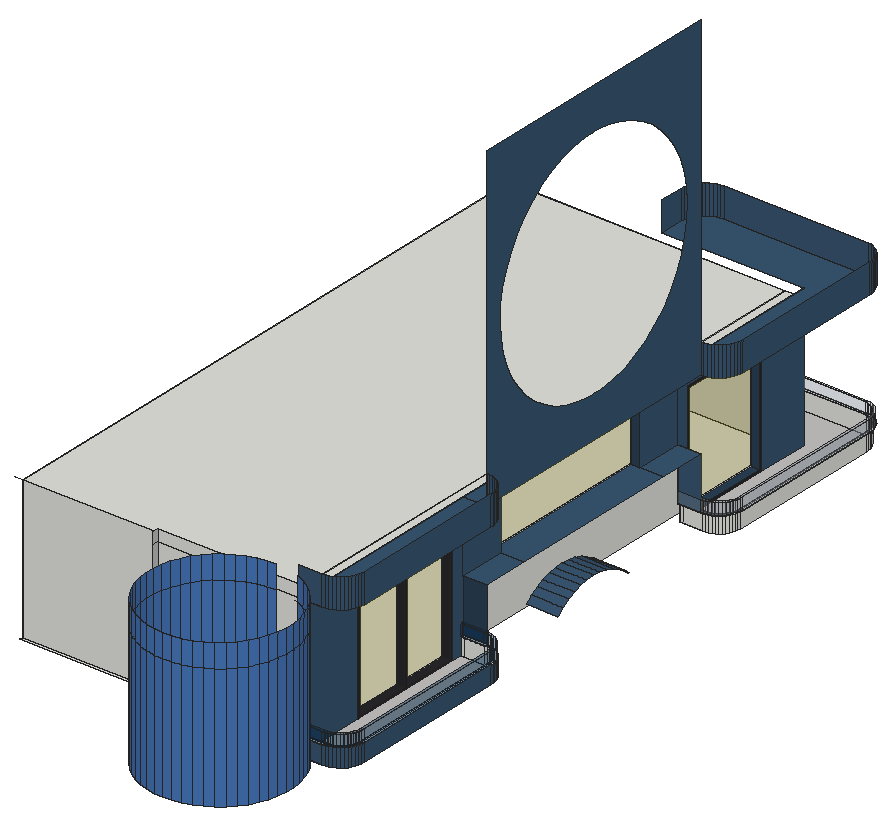
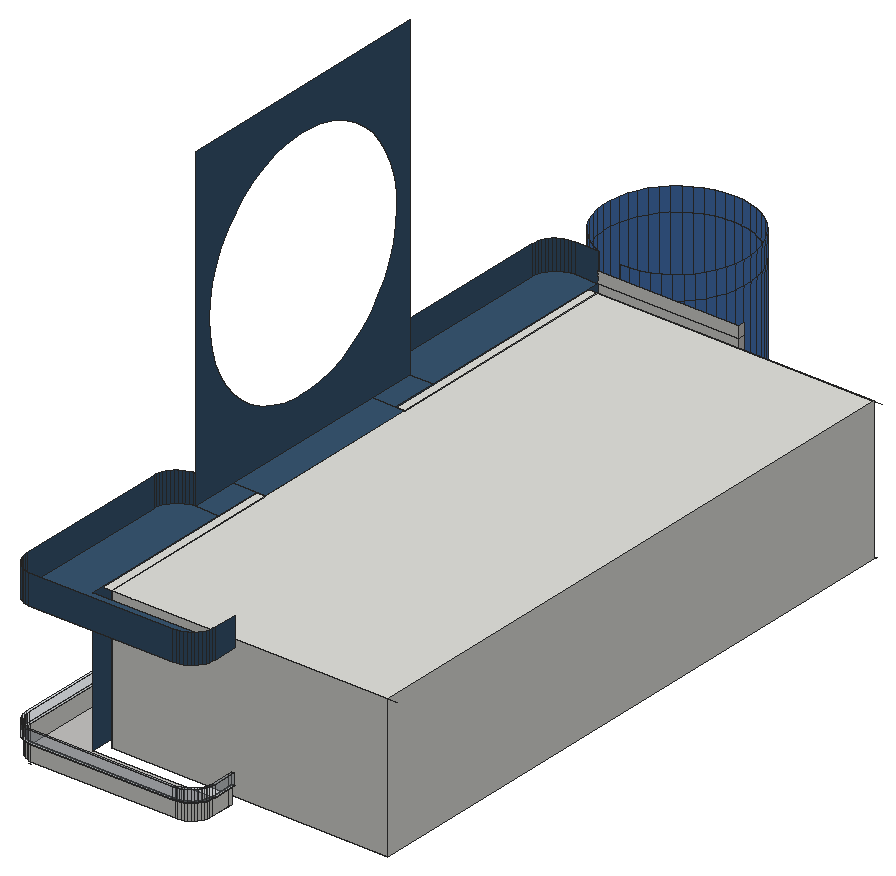
# SketchUp Ruby script. Lengths in inches.
U = 1.inch
M = Sketchup.active_model
def pt(a) = Geom::Point3d.new(a.map { |v| v * U })
def face(e, loops, mat)
  f = e.add_face(loops[0].map { |a| pt(a) })
  loops[1..].each { |l| e.add_face(l.map { |a| pt(a) }).erase! }
  f.material = f.back_material = mat if mat
  f
end
# faces: each face lists its corners as indices into pts; further lists are holes
def faces(e, pts, list, mat = nil) = list.each { |f| face(e, (f[0].is_a?(Array) ? f : [f]).map { |l| l.map { |i| pts[i] } }, mat) }
# xy, xz, yz: faces in a plane at the given z, y or x. An outline is a flat list of corners, or four numbers for a rectangle; further outlines are holes
def ring(l) = l.size == 4 ? [[l[0], l[1]], [l[2], l[1]], [l[2], l[3]], [l[0], l[3]]] : l.each_slice(2).to_a
def flat(e, list, mat, &to3) = list.each { |f| face(e, (f[0].is_a?(Array) ? f : [f]).map { |l| ring(l).map { |u, v| to3.(u, v) } }, mat) }
def xy(e, z, list, mat = nil) = flat(e, list, mat) { |x, y| [x, y, z] }
def xz(e, y, list, mat = nil) = flat(e, list, mat) { |x, z| [x, y, z] }
def yz(e, x, list, mat = nil) = flat(e, list, mat) { |y, z| [x, y, z] }
def lines(e, pts, list) = list.each { |a, b| e.add_line(pt(pts[a]), pt(pts[b])) }
# prism: a flat outline (further loops are holes) pulled along v
def prism(e, loops, v, mat = nil)
  f = face(e, loops, mat); d = Geom::Vector3d.new(v.map { |x| x * U })
  f.pushpull(f.normal.samedirection?(d) ? d.length : -d.length)
end
def box(e, o, s, mat = nil) = prism(e, [[o, [o[0] + s[0], o[1], o[2]], [o[0] + s[0], o[1] + s[1], o[2]], [o[0], o[1] + s[1], o[2]]]], [0, 0, s[2]], mat)
def at(x, y, z, deg = 0) = Geom::Transformation.translation(pt([x, y, z])) * Geom::Transformation.rotation(ORIGIN, Z_AXIS, deg.degrees)
def axes(o, x, y, z) = Geom::Transformation.new([*x, 0, *y, 0, *z, 0, *pt(o).to_a, 1])
def part(name) = M.definitions.add(name)
# library, detail: a bought-in or finely detailed component or shape, given as its bounding box
def library(name, o, s) = part(name).tap { |d| box(d.entities, o, s) }
def detail(e, o, s) = box(e.add_group.entities, o, s)
def put(e, d, t, mat = nil) = e.add_instance(d, t).tap { |i| i.material = mat if mat }
def group(e, t, mat = nil) = e.add_group.tap { |g| g.transformation = t; g.material = mat if mat }.entities
root = M.entities
M.materials.add("Carpet_01_1K").color = [196, 195, 193]
M.materials.add("Carpet_04_1K").color = [56, 85, 112]
M.materials.add("Carpet_04_1K1").color = [43, 65, 85]
M.materials.add("Glass_Basic_01").color = [186, 175, 28]
M.materials["Glass_Basic_01"].alpha = 0.25
M.materials.add("Glass_Basic_1").color = [0, 47, 91]
M.materials["Glass_Basic_1"].alpha = 0.25
M.materials.add("Glass_Basic_2").color = [161, 173, 186]
M.materials["Glass_Basic_2"].alpha = 0.25
M.materials.add("Glass_Mirror_01").color = [71, 118, 185]
M.materials.add("ThomThom - Buttons2").color = [40, 40, 43]
c1 = part("Group\#1")
prism(c1.entities,[[[0,206.04,0],[0,209.04,0],[24,209.04,0],[24.001,209.04,0],[27.133,208.835,0],[30.212,208.222,0],[33.184,207.213,0],[36,205.825,0],[38.61,204.081,0],[40.971,202.011,0],[43.04,199.65,0],[44.785,197.04,0],[46.173,194.224,0],[47.182,191.252,0],[47.795,188.173,0],[48,185.04,0],[48,24,0],[47.795,20.867,0],[47.182,17.788,0],[46.602,16.08,0],[46.173,14.816,0],[44.785,12,0],[43.04,9.39,0],[40.971,7.029,0],[38.61,4.96,0],[36,3.215,0],[33.184,1.827,0],[30.212,0.818,0],[27.133,0.205,0],[24,0,0],[0,0,0],[0,3,0],[3,3,0],[24,3,0],[26.741,3.18,0],[29.435,3.716,0],[32.036,4.599,0],[34.5,5.814,0],[36.784,7.34,0],[38.849,9.151,0],[40.66,11.216,0],[42.187,13.5,0],[43.401,15.964,0],[44.284,18.565,0],[44.82,21.259,0],[45,24,0],[45,185.04,0],[44.82,187.781,0],[44.284,190.475,0],[43.401,193.076,0],[42.187,195.54,0],[40.66,197.824,0],[38.849,199.889,0],[36.784,201.701,0],[34.5,203.227,0],[32.036,204.442,0],[29.435,205.325,0],[26.741,205.86,0],[24,206.04,0],[3,206.04,0]]],[0,0,12])
c2 = part("Group\#2")
prism(c2.entities,[[[147,3,0],[168,3,0],[170.74,3.18,0],[173.44,3.72,0],[176.04,4.6,0],[178.5,5.8125,0],[180.78,7.34,0],[182.85,9.15,0],[184.66,11.22,0],[186.1875,13.5,0],[187.4,15.96,0],[188.28,18.56,0],[188.82,21.26,0],[189,24,0],[189,184.94,0],[188.8125,187.78,0],[188.28,190.47,0],[187.4,193.07,0],[186.18,195.54,0],[184.66,197.82,0],[182.84,199.88,0],[180.78,201.7,0],[178.5,203.22,0],[176.03,204.4375,0],[173.43,205.32,0],[171.01,205.8,0],[24,205.8,0],[21.26,205.62,0],[18.56,205.08,0],[15.96,204.2,0],[13.5,202.99,0],[11.22,201.46,0],[9.15,199.65,0],[7.34,197.58,0],[5.8125,195.3,0],[4.6,192.84,0],[3.72,190.24,0],[3.18,187.54,0],[3,184.8,0],[3,163.8,0],[3,160.8,0],[0,160.8,0],[0,184.8,0],[0.21,187.93,0],[0.82,191.01,0],[1.83,193.98,0],[3.22,196.8,0],[4.96,199.41,0],[7.03,201.77,0],[9.39,203.84,0],[12,205.58,0],[14.82,206.97,0],[17.79,207.98,0],[20.87,208.59,0],[24,208.8,0],[171.31,208.8,0],[174.21,208.22,0],[177.18,207.21,0],[180,205.82,0],[182.61,204.08,0],[184.97,202.01,0],[187.04,199.65,0],[188.78,197.04,0],[190.17,194.22,0],[191.18,191.25,0],[191.79,188.17,0],[192,185.04,0],[192,24,0],[191.79,20.87,0],[191.18,17.79,0],[190.17,14.82,0],[188.78,12,0],[187.04,9.39,0],[184.97,7.03,0],[182.61,4.96,0],[180,3.22,0],[177.18,1.83,0],[174.21,0.82,0],[171.13,0.21,0],[168,0,0],[144,0,0],[144,3,0]]],[0,0,12])
xy(root,461.77,[[330.57,155.5,354.57,155.5,357.71,155.71,360.79,156.32,363.76,157.33,366.57,158.72,369.19,160.46,371.55,162.53,373.62,164.89,375.36,167.5,376.75,170.32,377.76,173.29,378.37,176.37,378.57,179.5,378.57,340.54,378.37,343.67,377.76,346.75,376.75,349.73,375.36,352.54,373.62,355.15,371.55,357.51,369.19,359.58,366.57,361.33,363.76,362.71,360.79,363.72,357.71,364.34,354.58,364.54,330.57,364.54,330.57,361.54,354.57,361.54,357.32,361.36,360.01,360.83,362.61,359.94,365.07,358.73,367.36,357.2,369.42,355.39,371.24,353.33,372.76,351.04,373.98,348.58,374.86,345.98,375.4,343.28,375.57,340.54,375.57,179.5,375.4,176.76,374.86,174.07,373.98,171.46,372.76,169,371.24,166.72,369.42,164.65,367.36,162.84,365.07,161.31,362.61,160.1,360.01,159.22,357.32,158.68,354.57,158.5,330.57,158.5]])
xy(root,462,[[39.57,164.5,321.57,167.5625],[39.57,167.5625,321.57,786.64]])
xy(root,462,[[330.57,158.5,354.57,158.5,357.32,158.68,360.01,159.22,362.61,160.1,365.07,161.31,367.36,162.84,369.42,164.65,371.24,166.72,372.76,169,373.98,171.46,374.86,174.07,375.4,176.76,375.57,179.5,375.57,340.54,375.4,343.28,374.86,345.98,373.98,348.58,372.76,351.04,371.24,353.33,369.42,355.39,367.36,357.2,365.07,358.73,362.61,359.94,360.01,360.83,357.32,361.36,354.57,361.54,330.57,361.54],[330.57,640.9,354.57,640.9,357.32,641.08,360.01,641.62,362.61,642.5,365.07,643.71,367.36,645.24,369.42,647.05,371.24,649.12,372.76,651.4,373.98,653.86,374.86,656.47,375.4,659.16,375.57,661.9,375.57,822.84,375.39,825.68,374.85,828.375,373.97,830.97,372.76,833.4375,371.23,835.72,369.42,837.79,367.36,839.6,365.07,841.12,362.61,842.34,360.01,843.22,357.59,843.7,210.57,843.7,207.83,843.52,205.14,842.99,202.54,842.1,200.07,840.89,197.79,839.36,195.73,837.55,193.91,835.48,192.39,833.2,191.17,830.74,190.29,828.14,189.75,825.44,189.57,822.7,189.57,798.7,330.57,798.7]],"Carpet_01_1K")
xy(root,463.77,[[321.57,233.15,330.57,291.15],[321.57,293.15,330.57,349.15]],"ThomThom - Buttons2")
xy(root,465,[[321.57,652.9,330.57,742.9]],"Carpet_04_1K1")
xy(root,480,[[330.57,155.5,354.57,155.5,357.71,155.71,360.79,156.32,363.76,157.33,366.57,158.72,369.19,160.46,371.55,162.53,373.62,164.89,375.36,167.5,376.75,170.32,377.76,173.29,378.37,176.37,378.57,179.5,378.57,340.54,378.37,343.67,377.76,346.75,376.75,349.73,375.36,352.54,373.62,355.15,371.55,357.51,369.19,359.58,366.57,361.33,363.76,362.71,360.79,363.72,357.71,364.34,354.58,364.54,330.57,364.54,330.57,361.54,354.57,361.54,357.32,361.36,360.01,360.83,362.61,359.94,365.07,358.73,367.36,357.2,369.42,355.39,371.24,353.33,372.76,351.04,373.98,348.58,374.86,345.98,375.4,343.28,375.57,340.54,375.57,179.5,375.4,176.76,374.86,174.07,373.98,171.46,372.76,169,371.24,166.72,369.42,164.65,367.36,162.84,365.07,161.31,362.61,160.1,360.01,159.22,357.32,158.68,354.57,158.5,330.57,158.5],[330.57,637.9,354.57,637.9,357.71,638.11,360.79,638.72,363.76,639.73,366.57,641.12,369.19,642.86,371.55,644.93,373.62,647.29,375.36,649.9,376.75,652.72,377.76,655.6875,378.37,658.77,378.57,661.9,378.57,822.94,378.37,826.07,377.76,829.15,376.75,832.125,375.36,834.94,373.62,837.55,371.55,839.91,369.19,841.98,366.57,843.73,363.76,845.11,360.79,846.12,357.88,846.7,210.57,846.7,207.44,846.5,204.36,845.88,201.39,844.875,198.57,843.49,195.96,841.74,193.6,839.67,191.53,837.3125,189.79,834.7,188.4,831.89,187.39,828.91,186.78,825.83,186.57,822.7,186.57,798.7,189.57,798.7,189.57,822.7,189.75,825.44,190.29,828.14,191.17,830.74,192.39,833.2,193.91,835.48,195.73,837.55,197.79,839.36,200.07,840.89,202.54,842.1,205.14,842.99,207.83,843.52,210.57,843.7,357.59,843.7,360.01,843.22,362.61,842.34,365.07,841.12,367.36,839.6,369.42,837.79,371.23,835.72,372.76,833.4375,373.97,830.97,374.85,828.375,375.39,825.68,375.57,822.84,375.57,661.9,375.4,659.16,374.86,656.47,373.98,653.86,372.76,651.4,371.24,649.12,369.42,647.05,367.36,645.24,365.07,643.71,362.61,642.5,360.01,641.62,357.32,641.08,354.57,640.9,330.57,640.9]])
xy(root,483,[[322.57,501.22,354.57,501.27]],"Carpet_04_1K")
xy(root,534,[[330.57,364.54,354.57,412.54],[321.57,412.54,354.57,589.9],[330.57,589.9,354.57,637.9]],"Carpet_04_1K")
xy(root,579,[[321.57,652.9,330.57,742.9]],"Carpet_04_1K1")
xy(root,585.77,[[321.57,233.15,330.57,291.15],[321.57,293.15,330.57,349.15]],"ThomThom - Buttons2")
xy(root,606,[[39.57,167.5625,321.57,786.64],[321.57,167.5625,330.57,412.54],[321.57,589.9,330.57,786.64]])
xy(root,606,[[330.57,155.5,330.57,364.54,354.57,364.54,357.71,364.34,360.79,363.72,363.76,362.71,366.57,361.33,369.19,359.58,371.55,357.51,373.62,355.15,375.36,352.54,376.75,349.73,377.76,346.75,378.37,343.67,378.57,340.54,378.57,179.5,378.37,176.37,377.76,173.29,376.75,170.32,375.36,167.5,373.62,164.89,371.55,162.53,369.19,160.46,366.57,158.72,363.76,157.33,360.79,156.32,357.71,155.71,354.57,155.5],[330.57,364.54,354.57,412.54],[321.57,412.54,354.57,589.9],[330.57,589.9,354.57,637.9],[330.57,637.9,330.57,798.7,186.57,798.7,186.57,822.7,186.78,825.83,187.39,828.91,188.4,831.89,189.79,834.7,191.53,837.3125,193.6,839.67,195.96,841.74,198.57,843.49,201.39,844.875,204.36,845.88,207.44,846.5,210.57,846.7,357.88,846.7,360.79,846.12,363.76,845.11,366.57,843.73,369.19,841.98,371.55,839.91,373.62,837.55,375.36,834.94,376.75,832.125,377.76,829.15,378.37,826.07,378.57,822.94,378.57,661.9,378.37,658.77,377.76,655.6875,376.75,652.72,375.36,649.9,373.62,647.29,371.55,644.93,369.19,642.86,366.57,641.12,363.76,639.73,360.79,638.72,357.71,638.11,354.57,637.9]],"Carpet_04_1K")
xz(root,155.5,[[186.57,462,330.57,606],[186.57,606,330.57,618]])
xz(root,155.5,[[330.57,461.77,354.57,480],[330.57,606,354.57,636]],"Carpet_04_1K")
xz(root,158.5,[[330.57,462,333.57,480],[333.57,462,354.57,480]])
xz(root,167.5625,[[39.57,462,321.57,606]])
xz(root,233.15,[[321.57,463.77,330.57,585.77]],"ThomThom - Buttons2")
xz(root,291.15,[[321.57,463.77,330.57,585.77]],"ThomThom - Buttons2")
xz(root,293.15,[[321.57,463.77,330.57,585.77]])
xz(root,349.15,[[321.57,463.77,330.57,585.77]],"ThomThom - Buttons2")
xz(root,361.54,[[330.57,462,333.57,480],[333.57,462,354.57,480]])
xz(root,364.54,[[354.57,461.77,354.58,480]])
xz(root,364.54,[[330.57,480,354.57,534]],"Carpet_04_1K1")
xz(root,412.54,[[321.57,534,330.57,606]])
xz(root,589.9,[[321.57,534,330.57,606]],"Carpet_04_1K1")
xz(root,637.9,[[330.57,480,354.57,534]],"Carpet_04_1K")
xz(root,640.9,[[330.57,462,333.57,480],[333.57,462,354.57,480]])
xz(root,652.9,[[321.57,465,330.57,579]])
xz(root,742.9,[[321.57,465,330.57,579]],"Carpet_04_1K1")
xz(root,786.64,[[39.57,462,321.57,606]])
xz(root,843.7,[[210.57,462,357.59,480]])
xz(root,846.7,[[210.57,606,357.88,636]],"Carpet_04_1K")
yz(root,39.57,[[167.5625,462,786.64,606]])
yz(root,186.57,[[149.51,462,155.5,606],[149.51,606,155.5,618]],"Carpet_01_1K")
yz(root,186.57,[[798.7,606,822.7,636]],"Carpet_04_1K")
yz(root,189.57,[[798.7,462,801.7,480],[801.7,462,822.7,480]])
yz(root,236.92,[[77.22,480,86.26,606],[77.22,606,86.26,630]],"Glass_Mirror_01")
yz(root,321.57,[[[167.5625,462,167.5625,606,412.54,606,412.54,534,589.9,534,589.9,606,786.64,606,786.64,462],[652.9,465,742.9,579],[233.15,463.77,291.15,585.77],[293.15,463.77,349.15,585.77]]])
yz(root,321.57,[[233.15,463.77,291.15,585.77],[293.15,463.77,349.15,585.77],[652.9,465,742.9,579],[412.54,534,589.9,606]],"Glass_Basic_01")
yz(root,330.57,[[231.15,461.77,351.15,462]])
yz(root,330.57,[[158.5,462,231.15,462,231.15,587.77,351.15,587.77,351.15,462,361.54,462,361.54,480,364.54,480,364.54,606,155.5,606,155.5,480,158.5,480],[640.9,462,649.9,462,649.9,582,745.9,582,745.9,462,798.7,462,798.7,606,637.9,606,637.9,480,640.9,480],[364.54,534,412.54,606],[589.9,534,637.9,606]],"Carpet_04_1K")
yz(root,330.57,[[[231.15,462,351.15,587.77],[233.15,463.77,233.15,585.77,349.15,585.77,349.15,463.77,293.15,463.77,293.15,585.77,291.15,585.77,291.15,463.77]],[649.9,462,652.9,462,652.9,579,745.9,579,745.9,582,649.9,582],[652.9,462,745.9,462,745.9,579,742.9,579,742.9,465,652.9,465]],"ThomThom - Buttons2")
yz(root,354.57,[[[364.54,606,637.9,930],[495.8125,648.12,480.83,649.75,466.17,653.23,452.0625,658.53,438.73,665.56,426.38,674.2,415.22,684.32,405.41,695.75,397.11,708.33,390.45,721.85,385.54,736.1,382.45,750.85,381.24,765.87,381.92,780.93,384.48,795.78,388.88,810.1875,395.06,823.9375,402.9,836.8,412.3,848.58,423.1,859.09,435.13,868.16,448.21,875.66,462.12,881.45,476.65,885.46,491.5625,887.61,501.22,887.78,506.63,887.88,521.61,886.25,536.27,882.77,550.38,877.47,563.71,870.44,576.06,861.8,587.23,851.68,597.04,840.25,605.34,827.67,611.99,814.15,616.9,799.9,619.99,785.15,621.2,770.13,620.52,755.07,617.96,740.22,613.56,725.8125,607.39,712.0625,599.54,699.2,590.14,687.42,579.34,676.91,567.31,667.84,554.23,660.34,540.32,654.55,525.79,650.54,510.88,648.39,501.22,648.22]]],"Carpet_04_1K")
yz(root,375.57,[[179.5,462,340.54,480],[661.9,462,822.84,480]])
yz(root,378.57,[[179.5,461.77,340.54,480],[179.5,606,340.54,636],[661.9,606,822.94,636]],"Carpet_04_1K")
yz(root,380.64,[[77.22,480,86.26,606],[77.22,606,86.26,630]],"Glass_Mirror_01")
p = [[354.57,155.5,480],[354.57,155.5,461.77],[357.71,155.71,461.77],[357.71,155.71,480],[360.79,156.32,461.77],[360.79,156.32,480],
  [363.76,157.33,461.77],[363.76,157.33,480],[366.57,158.72,461.77],[366.57,158.72,480],[369.19,160.46,461.77],[369.19,160.46,480],
  [371.55,162.53,461.77],[371.55,162.53,480],[373.62,164.89,461.77],[373.62,164.89,480],[375.36,167.5,461.77],[375.36,167.5,480],
  [376.75,170.32,461.77],[376.75,170.32,480],[377.76,173.29,461.77],[377.76,173.29,480],[378.37,176.37,461.77],[378.37,176.37,480],
  [378.57,179.5,461.77],[378.57,179.5,480],[378.57,340.54,480],[378.57,340.54,461.77],[378.37,343.67,461.77],[378.37,343.67,480],
  [377.76,346.75,461.77],[377.76,346.75,480],[376.75,349.73,461.77],[376.75,349.73,480],[375.36,352.54,461.77],[375.36,352.54,480],
  [373.62,355.15,461.77],[373.62,355.15,480],[371.55,357.51,461.77],[371.55,357.51,480],[369.19,359.58,461.77],[369.19,359.58,480],
  [366.57,361.33,461.77],[366.57,361.33,480],[363.76,362.71,461.77],[363.76,362.71,480],[360.79,363.72,461.77],[360.79,363.72,480],
  [357.71,364.34,461.77],[357.71,364.34,480],[354.58,364.54,461.77],[354.58,364.54,480],[357.32,158.68,462],[354.57,158.5,462],
  [354.57,158.5,480],[357.32,158.68,480],[360.01,159.22,462],[360.01,159.22,480],[362.61,160.1,462],[362.61,160.1,480],
  [365.07,161.31,462],[365.07,161.31,480],[367.36,162.84,462],[367.36,162.84,480],[369.42,164.65,462],[369.42,164.65,480],
  [371.24,166.72,462],[371.24,166.72,480],[372.76,169,462],[372.76,169,480],[373.98,171.46,462],[373.98,171.46,480],
  [374.86,174.07,462],[374.86,174.07,480],[375.4,176.76,462],[375.4,176.76,480],[375.57,179.5,462],[375.57,179.5,480],
  [375.4,343.28,462],[375.57,340.54,462],[375.57,340.54,480],[375.4,343.28,480],[374.86,345.98,462],[374.86,345.98,480],
  [373.98,348.58,462],[373.98,348.58,480],[372.76,351.04,462],[372.76,351.04,480],[371.24,353.33,462],[371.24,353.33,480],
  [369.42,355.39,462],[369.42,355.39,480],[367.36,357.2,462],[367.36,357.2,480],[365.07,358.73,462],[365.07,358.73,480],
  [362.61,359.94,462],[362.61,359.94,480],[360.01,360.83,462],[360.01,360.83,480],[357.32,361.36,462],[357.32,361.36,480],
  [354.57,361.54,462],[354.57,361.54,480],[357.32,641.08,462],[354.57,640.9,462],[354.57,640.9,480],[357.32,641.08,480],
  [360.01,641.62,462],[360.01,641.62,480],[362.61,642.5,462],[362.61,642.5,480],[365.07,643.71,462],[365.07,643.71,480],
  [367.36,645.24,462],[367.36,645.24,480],[369.42,647.05,462],[369.42,647.05,480],[371.24,649.12,462],[371.24,649.12,480],
  [372.76,651.4,462],[372.76,651.4,480],[373.98,653.86,462],[373.98,653.86,480],[374.86,656.47,462],[374.86,656.47,480],
  [375.4,659.16,462],[375.4,659.16,480],[375.57,661.9,462],[375.57,661.9,480],[189.57,822.7,462],[189.75,825.44,462],
  [189.75,825.44,480],[189.57,822.7,480],[375.39,825.68,462],[375.57,822.84,462],[375.57,822.84,480],[375.39,825.68,480],
  [190.29,828.14,462],[190.29,828.14,480],[374.85,828.375,462],[374.85,828.375,480],[191.17,830.74,462],[191.17,830.74,480],
  [373.97,830.97,462],[373.97,830.97,480],[192.39,833.2,462],[192.39,833.2,480],[372.76,833.4375,462],[372.76,833.4375,480],
  [193.91,835.48,462],[193.91,835.48,480],[371.23,835.72,462],[371.23,835.72,480],[195.73,837.55,462],[195.73,837.55,480],
  [369.42,837.79,462],[369.42,837.79,480],[197.79,839.36,462],[197.79,839.36,480],[367.36,839.6,462],[367.36,839.6,480],
  [200.07,840.89,462],[200.07,840.89,480],[365.07,841.12,462],[365.07,841.12,480],[202.54,842.1,462],[202.54,842.1,480],
  [362.61,842.34,462],[362.61,842.34,480],[205.14,842.99,462],[205.14,842.99,480],[360.01,843.22,462],[360.01,843.22,480],
  [207.83,843.52,462],[207.83,843.52,480],[357.59,843.7,462],[357.59,843.7,480],[210.57,843.7,462],[210.57,843.7,480],
  [322.57,462.47,470.43],[354.57,462.47,470.43],[354.57,456.08,465.15],[322.57,456.08,465.15],[322.57,546.4375,465.08],[354.57,546.4375,465.08],
  [354.57,540.06,470.36],[322.57,540.06,470.36],[322.57,469.47,474.86],[354.57,469.47,474.86],[354.57,533.0625,474.8125],[322.57,533.0625,474.8125],
  [354.57,525.57,478.35],[322.57,525.57,478.35],[322.57,476.97,478.38],[354.57,476.97,478.38],[354.57,517.68,480.91],[322.57,517.68,480.91],
  [322.57,484.86,480.9375],[354.57,484.86,480.9375],[299.76,10.31,606],[299.76,10.31,480],[308.78,9.74,480],[308.78,9.74,606],
  [317.8,10.31,480],[317.8,10.31,606],[290.875,12,606],[290.875,12,480],[326.6875,12,480],[326.6875,12,606],
  [282.28,14.79,606],[282.28,14.79,480],[335.29,14.79,480],[335.29,14.79,606],[274.09,18.64,606],[274.09,18.64,480],
  [343.47,18.64,480],[343.47,18.64,606],[266.46,23.49,606],[266.46,23.49,480],[351.1,23.49,480],[351.1,23.49,606],
  [259.49,29.25,606],[259.49,29.25,480],[358.07,29.25,480],[358.07,29.25,606],[253.3,35.84,606],[253.3,35.84,480],
  [364.26,35.84,480],[364.26,35.84,606],[247.99,43.16,606],[247.99,43.16,480],[369.57,43.16,480],[369.57,43.16,606],
  [243.63,51.08,606],[243.63,51.08,480],[373.93,51.08,480],[373.93,51.08,606],[240.3,59.49,606],[240.3,59.49,480],
  [377.26,59.49,480],[377.26,59.49,606],[238.06,68.25,606],[238.06,68.25,480],[379.51,68.25,480],[379.51,68.25,606],
  [236.92,77.22,606],[236.92,77.22,480],[380.64,77.22,480],[380.64,77.22,606],[238.06,95.23,606],[238.06,95.23,480],
  [236.92,86.26,480],[236.92,86.26,606],[380.64,86.26,606],[380.64,86.26,480],[379.51,95.23,480],[379.51,95.23,606],
  [240.3,103.99,606],[240.3,103.99,480],[377.26,103.99,480],[377.26,103.99,606],[243.63,112.39,606],[243.63,112.39,480],
  [373.93,112.39,480],[373.93,112.39,606],[247.99,120.32,606],[247.99,120.32,480],[369.57,120.32,480],[369.57,120.32,606],
  [253.3,127.63,606],[253.3,127.63,480],[364.26,127.63,480],[364.26,127.63,606],[259.49,134.22,606],[259.49,134.22,480],
  [358.07,134.22,480],[358.07,134.22,606],[266.46,139.99,606],[266.46,139.99,480],[351.1,139.99,480],[351.1,139.99,606],
  [274.09,144.83,606],[274.09,144.83,480],[343.47,144.83,480],[343.47,144.83,606],[282.28,148.68,606],[282.28,148.68,480],
  [335.29,148.68,480],[335.29,148.68,606],[290.875,151.48,606],[290.875,151.48,480],[299.76,153.17,606],[299.76,153.17,480],
  [308.78,153.74,606],[308.78,153.74,480],[322.57,493,482.49],[354.57,493,482.49],[354.57,509.54,482.47],[322.57,509.54,482.47],
  [322.57,501.22,483],[354.57,501.22,483],[354.57,501.27,483],[322.57,501.27,483],[308.78,9.74,630],[299.76,10.31,630],
  [317.8,10.31,630],[290.875,12,630],[326.6875,12,630],[282.28,14.79,630],[335.29,14.79,630],[274.09,18.64,630],
  [343.47,18.64,630],[266.46,23.49,630],[351.1,23.49,630],[259.49,29.25,630],[358.07,29.25,630],[253.3,35.84,630],
  [364.26,35.84,630],[247.99,43.16,630],[369.57,43.16,630],[243.63,51.08,630],[373.93,51.08,630],[240.3,59.49,630],
  [377.26,59.49,630],[238.06,68.25,630],[379.51,68.25,630],[236.92,77.22,630],[380.64,77.22,630],[236.92,86.26,630],
  [238.06,95.23,630],[379.51,95.23,630],[380.64,86.26,630],[240.3,103.99,630],[377.26,103.99,630],[243.63,112.39,630],
  [373.93,112.39,630],[247.99,120.32,630],[369.57,120.32,630],[253.3,127.63,630],[364.26,127.63,630],[259.49,134.22,630],
  [358.07,134.22,630],[266.46,139.99,630],[351.1,139.99,630],[274.09,144.83,630],[343.47,144.83,630],[282.28,148.68,630],
  [335.29,148.68,630],[290.875,151.48,630],[299.76,153.17,630],[308.78,153.74,630],[357.71,155.71,606],[357.71,155.71,636],
  [354.57,155.5,636],[354.57,155.5,606],[360.79,156.32,606],[360.79,156.32,636],[363.76,157.33,606],[363.76,157.33,636],
  [366.57,158.72,606],[366.57,158.72,636],[369.19,160.46,606],[369.19,160.46,636],[371.55,162.53,606],[371.55,162.53,636],
  [373.62,164.89,606],[373.62,164.89,636],[375.36,167.5,606],[375.36,167.5,636],[376.75,170.32,606],[376.75,170.32,636],
  [377.76,173.29,606],[377.76,173.29,636],[378.37,176.37,606],[378.37,176.37,636],[378.57,179.5,606],[378.57,179.5,636],
  [378.37,343.67,606],[378.37,343.67,636],[378.57,340.54,636],[378.57,340.54,606],[377.76,346.75,606],[377.76,346.75,636],
  [376.75,349.73,606],[376.75,349.73,636],[375.36,352.54,606],[375.36,352.54,636],[373.62,355.15,606],[373.62,355.15,636],
  [371.55,357.51,606],[371.55,357.51,636],[369.19,359.58,606],[369.19,359.58,636],[366.57,361.33,606],[366.57,361.33,636],
  [363.76,362.71,606],[363.76,362.71,636],[360.79,363.72,606],[360.79,363.72,636],[357.71,364.34,606],[357.71,364.34,636],
  [354.57,364.54,606],[354.57,364.54,636],[357.71,638.11,606],[357.71,638.11,636],[354.57,637.9,636],[354.57,637.9,606],
  [360.79,638.72,606],[360.79,638.72,636],[363.76,639.73,606],[363.76,639.73,636],[366.57,641.12,606],[366.57,641.12,636],
  [369.19,642.86,606],[369.19,642.86,636],[371.55,644.93,606],[371.55,644.93,636],[373.62,647.29,606],[373.62,647.29,636],
  [375.36,649.9,606],[375.36,649.9,636],[376.75,652.72,606],[376.75,652.72,636],[377.76,655.6875,606],[377.76,655.6875,636],
  [378.37,658.77,606],[378.37,658.77,636],[378.57,661.9,606],[378.57,661.9,636],[186.57,822.7,606],[186.57,822.7,636],
  [186.78,825.83,636],[186.78,825.83,606],[378.37,826.07,606],[378.37,826.07,636],[378.57,822.94,636],[378.57,822.94,606],
  [187.39,828.91,636],[187.39,828.91,606],[377.76,829.15,606],[377.76,829.15,636],[188.4,831.89,636],[188.4,831.89,606],
  [376.75,832.125,606],[376.75,832.125,636],[189.79,834.7,636],[189.79,834.7,606],[375.36,834.94,606],[375.36,834.94,636],
  [191.53,837.3125,636],[191.53,837.3125,606],[373.62,837.55,606],[373.62,837.55,636],[193.6,839.67,636],[193.6,839.67,606],
  [371.55,839.91,606],[371.55,839.91,636],[195.96,841.74,636],[195.96,841.74,606],[369.19,841.98,606],[369.19,841.98,636],
  [198.57,843.49,636],[198.57,843.49,606],[366.57,843.73,606],[366.57,843.73,636],[201.39,844.875,636],[201.39,844.875,606],
  [363.76,845.11,606],[363.76,845.11,636],[204.36,845.88,636],[204.36,845.88,606],[360.79,846.12,606],[360.79,846.12,636],
  [207.44,846.5,636],[207.44,846.5,606],[357.88,846.7,618],[357.88,846.7,636],[357.88,846.7,606],[210.57,846.7,636],
  [210.57,846.7,606],[39.57,786.64,606],[30.57,786.64,606],[39.57,167.5625,606],[30.57,167.5625,606],[357.71,846.74,462],
  [354.57,846.94,462],[357.88,846.7,462],[330.57,150.21,606],[330.57,150.21,480]]
faces(root,p,[[0,1,2,3],[3,2,4,5],[5,4,6,7],[7,6,8,9],[9,8,10,11],[11,10,12,13],[13,12,14,15],[15,14,16,17],
  [17,16,18,19],[19,18,20,21],[21,20,22,23],[23,22,24,25],[26,27,28,29],[29,28,30,31],[31,30,32,33],[33,32,34,35],
  [35,34,36,37],[37,36,38,39],[39,38,40,41],[41,40,42,43],[43,42,44,45],[45,44,46,47],[47,46,48,49],[49,48,50,51],
  [180,181,182,183],[184,185,186,187],[188,189,181,180],[187,186,190,191],[191,190,192,193],[194,195,189,188],[193,192,196,197],[198,199,195,194],
  [296,297,199,198],[197,196,298,299],[300,301,297,296],[299,298,302,303],[352,353,354,355],[356,357,353,352],[358,359,357,356],[360,361,359,358],
  [362,363,361,360],[364,365,363,362],[366,367,365,364],[368,369,367,366],[370,371,369,368],[372,373,371,370],[374,375,373,372],[376,377,375,374],
  [378,379,380,381],[382,383,379,378],[384,385,383,382],[386,387,385,384],[388,389,387,386],[390,391,389,388],[392,393,391,390],[394,395,393,392],
  [396,397,395,394],[398,399,397,396],[400,401,399,398],[402,403,401,400],[404,405,406,407],[408,409,405,404],[410,411,409,408],[412,413,411,410],
  [414,415,413,412],[416,417,415,414],[418,419,417,416],[420,421,419,418],[422,423,421,420],[424,425,423,422],[426,427,425,424],[428,429,427,426],
  [430,431,432,433],[434,435,436,437],[433,432,438,439],[440,441,435,434],[439,438,442,443],[444,445,441,440],[443,442,446,447],[448,449,445,444],
  [447,446,450,451],[452,453,449,448],[451,450,454,455],[456,457,453,452],[455,454,458,459],[460,461,457,456],[459,458,462,463],[464,465,461,460],
  [463,462,466,467],[468,469,465,464],[467,466,470,471],[472,473,469,468],[471,470,474,475],[476,477,473,472,478],[475,474,479,480]],"Carpet_04_1K")
faces(root,p,[[52,53,54,55],[56,52,55,57],[58,56,57,59],[60,58,59,61],[62,60,61,63],[64,62,63,65],[66,64,65,67],[68,66,67,69],
  [70,68,69,71],[72,70,71,73],[74,72,73,75],[76,74,75,77],[78,79,80,81],[82,78,81,83],[84,82,83,85],[86,84,85,87],
  [88,86,87,89],[90,88,89,91],[92,90,91,93],[94,92,93,95],[96,94,95,97],[98,96,97,99],[100,98,99,101],[102,100,101,103],
  [104,105,106,107],[108,104,107,109],[110,108,109,111],[112,110,111,113],[114,112,113,115],[116,114,115,117],[118,116,117,119],[120,118,119,121],
  [122,120,121,123],[124,122,123,125],[126,124,125,127],[128,126,127,129],[130,131,132,133],[134,135,136,137],[131,138,139,132],[140,134,137,141],
  [138,142,143,139],[144,140,141,145],[142,146,147,143],[148,144,145,149],[146,150,151,147],[152,148,149,153],[150,154,155,151],[156,152,153,157],
  [154,158,159,155],[160,156,157,161],[158,162,163,159],[164,160,161,165],[162,166,167,163],[168,164,165,169],[166,170,171,167],[172,168,169,173],
  [170,174,175,171],[176,172,173,177],[174,178,179,175]])
faces(root,p,[[200,201,202,203],[203,202,204,205],[206,207,201,200],[205,204,208,209],[210,211,207,206],[209,208,212,213],[214,215,211,210],[213,212,216,217],
  [218,219,215,214],[217,216,220,221],[222,223,219,218],[221,220,224,225],[226,227,223,222],[225,224,228,229],[230,231,227,226],[229,228,232,233],
  [234,235,231,230],[233,232,236,237],[238,239,235,234],[237,236,240,241],[242,243,239,238],[241,240,244,245],[246,247,243,242],[245,244,248,249],
  [250,251,252,253],[254,255,256,257],[258,259,251,250],[257,256,260,261],[262,263,259,258],[261,260,264,265],[266,267,263,262],[265,264,268,269],
  [270,271,267,266],[269,268,272,273],[274,275,271,270],[273,272,276,277],[278,279,275,274],[277,276,280,281],[282,283,279,278],[281,280,284,285],
  [286,287,283,282],[285,284,288,289],[290,291,287,286],[292,293,291,290],[294,295,293,292],[203,304,305,200],[205,306,304,203],[200,305,307,206],
  [209,308,306,205],[206,307,309,210],[213,310,308,209],[210,309,311,214],[217,312,310,213],[214,311,313,218],[221,314,312,217],[218,313,315,222],
  [225,316,314,221],[222,315,317,226],[229,318,316,225],[226,317,319,230],[233,320,318,229],[230,319,321,234],[237,322,320,233],[234,321,323,238],
  [241,324,322,237],[238,323,325,242],[245,326,324,241],[242,325,327,246],[249,328,326,245],[253,329,330,250],[257,331,332,254],[250,330,333,258],
  [261,334,331,257],[258,333,335,262],[265,336,334,261],[262,335,337,266],[269,338,336,265],[266,337,339,270],[273,340,338,269],[270,339,341,274],
  [277,342,340,273],[274,341,343,278],[281,344,342,277],[278,343,345,282],[285,346,344,281],[282,345,347,286],[289,348,346,285],[286,347,349,290],
  [290,349,350,292],[292,350,351,294]],"Glass_Mirror_01")
lines(root,p,[[481,482],[483,484],[485,486],[487,485],[289,488],[288,489]])
put(root,c1,at(330.57,155.5,480),"Glass_Basic_1")
put(root,c2,at(186.57,637.9,480),"Glass_Basic_2")
